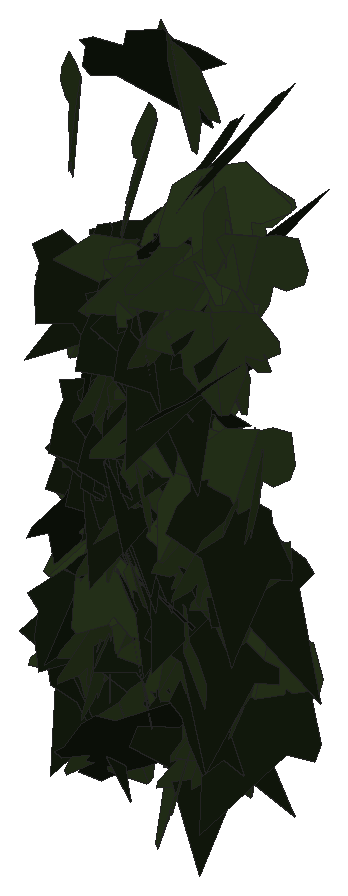
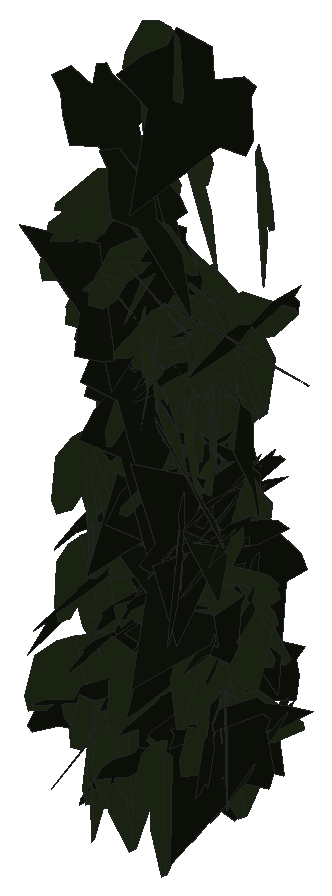
# SketchUp Ruby script. Lengths in inches.
U = 1.inch
M = Sketchup.active_model
def pt(a) = Geom::Point3d.new(a.map { |v| v * U })
def face(e, loops, mat)
  f = e.add_face(loops[0].map { |a| pt(a) })
  loops[1..].each { |l| e.add_face(l.map { |a| pt(a) }).erase! }
  f.material = f.back_material = mat if mat
  f
end
# faces: each face lists its corners as indices into pts; further lists are holes
def faces(e, pts, list, mat = nil) = list.each { |f| face(e, (f[0].is_a?(Array) ? f : [f]).map { |l| l.map { |i| pts[i] } }, mat) }
# xy, xz, yz: faces in a plane at the given z, y or x. An outline is a flat list of corners, or four numbers for a rectangle; further outlines are holes
def ring(l) = l.size == 4 ? [[l[0], l[1]], [l[2], l[1]], [l[2], l[3]], [l[0], l[3]]] : l.each_slice(2).to_a
def flat(e, list, mat, &to3) = list.each { |f| face(e, (f[0].is_a?(Array) ? f : [f]).map { |l| ring(l).map { |u, v| to3.(u, v) } }, mat) }
def xy(e, z, list, mat = nil) = flat(e, list, mat) { |x, y| [x, y, z] }
def xz(e, y, list, mat = nil) = flat(e, list, mat) { |x, z| [x, y, z] }
def yz(e, x, list, mat = nil) = flat(e, list, mat) { |y, z| [x, y, z] }
def lines(e, pts, list) = list.each { |a, b| e.add_line(pt(pts[a]), pt(pts[b])) }
# prism: a flat outline (further loops are holes) pulled along v
def prism(e, loops, v, mat = nil)
  f = face(e, loops, mat); d = Geom::Vector3d.new(v.map { |x| x * U })
  f.pushpull(f.normal.samedirection?(d) ? d.length : -d.length)
end
def box(e, o, s, mat = nil) = prism(e, [[o, [o[0] + s[0], o[1], o[2]], [o[0] + s[0], o[1] + s[1], o[2]], [o[0], o[1] + s[1], o[2]]]], [0, 0, s[2]], mat)
def at(x, y, z, deg = 0) = Geom::Transformation.translation(pt([x, y, z])) * Geom::Transformation.rotation(ORIGIN, Z_AXIS, deg.degrees)
def axes(o, x, y, z) = Geom::Transformation.new([*x, 0, *y, 0, *z, 0, *pt(o).to_a, 1])
def part(name) = M.definitions.add(name)
# library, detail: a bought-in or finely detailed component or shape, given as its bounding box
def library(name, o, s) = part(name).tap { |d| box(d.entities, o, s) }
def detail(e, o, s) = box(e.add_group.entities, o, s)
def put(e, d, t, mat = nil) = e.add_instance(d, t).tap { |i| i.material = mat if mat }
def group(e, t, mat = nil) = e.add_group.tap { |g| g.transformation = t; g.material = mat if mat }.entities
root = M.entities
M.materials.add("efeu1").color = [18, 25, 13]
M.materials.add("efeu2").color = [43, 57, 29]
c1 = part("ivyleaf_10")
p = [[0,0.5,-0.03],[-0.0625,2.02,-0.43],[-0.19,2.01,-0.46],[-0.54,1.05,-0.29],[-0.52,0.625,-0.18],[-0.83,0.76,-0.28],
  [-1.16,0.64,-0.33],[-1.15,0.33,-0.24],[-0.77,-0.39,0.02],[-0.3,-0.51,0.16],[0.04,-0.48,0.23],[-0.02,2.01,-0.4375],
  [-0.06,2.01,-0.43],[0.04,-0.49,0.23],[0.67,-0.49,0.14],[1.38,0.36,-0.2],[1.375,0.51,-0.24],[0.81,0.65,-0.19],
  [0.62,0.59,-0.15],[0.6,1.09,-0.28],[0.5,1.23,-0.31]]
faces(c1.entities,p,[[0,1,2,3,4,5,6,7,8,9,10],[11,12,0,13,14,15,16,17,18,19,20]],"efeu2")
c2 = part("ivyleaf_9")
p = [[1.54,2.16,1.25],[1.36,2.04,1.19],[-0.21,0.99,0.68],[-0.71,1.11,0.82],[-0.85,0.86,0.67],[-0.8,0.17,0.21],
  [-0.9,-0.01,0.1],[-0.67,-0.16,-0.02],[-0.08,-0.08,-0.05],[-0.03,-0.6,-0.4],[0.65,-0.88,-0.66],[0.83,-0.6,-0.49],
  [1.29,-0.42,-0.43],[1.8125,-0.07,-0.26],[1.21,0.44,0.15]]
faces(c2.entities,p,[[0,1,2,3,4,5,6,7,8,9,10,11,12,13,14]],"efeu1")
put(root,c1,axes([13.96,224.02,226.48],[-0.12869,-0.48261,0.02288],[-0.00453,-0.02247,-0.49947],[0.48313,-0.12876,0.00141]))
put(root,c2,axes([14.07,224.29,227.32],[-0.23689,-0.43392,0.07482],[0.01205,-0.09132,-0.49144],[0.44016,-0.23103,0.05372]))
put(root,c1,axes([14.31,223.89,230.38],[-0.44358,0.22112,0.06589],[-0.06998,0.00713,-0.49503],[-0.21986,-0.44839,0.02463]))
put(root,c1,axes([13.77,224.05,229.28],[0.28039,-0.4139,0.00816],[0.00734,-0.00488,-0.49992],[0.41392,0.28046,0.00334]))
put(root,c2,axes([13.1,224.04,227.85],[0.12777,-0.4541,-0.16573],[-0.03569,0.16209,-0.47165],[0.48208,0.13235,0.00901]))
put(root,c2,axes([13.4375,223.77,222.93],[0.23047,0.42069,-0.14108],[0.06968,0.12269,0.47968],[0.43821,-0.24077,-0.00207]))
put(root,c1,axes([14.66,223.95,227.68],[-0.41709,-0.27569,-0.00562],[0.0048,0.00294,-0.49997],[0.2757,-0.41712,0.00019]))
put(root,c1,axes([14.52,224.01,228.11],[-0.28727,-0.40846,0.02511],[-0.0115,-0.02262,-0.49936],[0.40907,-0.28748,0.0036]))
put(root,c1,axes([13.68,223.97,225.35],[-0.02424,-0.49206,-0.08536],[0.02223,0.08431,-0.49234],[0.49892,-0.02767,0.01779]))
put(root,c1,axes([13.62,223.91,224.78],[-0.2972,-0.28507,-0.28356],[0.29254,0.0886,-0.39569],[0.27584,-0.40111,0.11413]))
put(root,c2,axes([13.67,224.16,224.9],[-0.0708,0.26948,-0.41517],[0.0066,-0.41885,-0.27299],[-0.49492,-0.04413,0.05575]))
put(root,c1,axes([13.27,224.19,227.8125],[-0.16473,-0.43142,0.19169],[-0.02068,-0.19623,-0.45942],[0.47163,-0.15929,0.04681]))
put(root,c2,axes([13.44,224.35,225.83],[-0.17086,-0.45753,0.1071],[0.02661,-0.1232,-0.48385],[0.46915,-0.15964,0.06645]))
put(root,c2,axes([14.64,224.3,225.54],[0.00782,-0.49015,0.09847],[0.02788,-0.0979,-0.48953],[0.49916,0.01314,0.0258]))
put(root,c2,axes([13.74,224.24,227.85],[-0.49927,0.01901,0.01929],[-0.02354,-0.12868,-0.48258],[-0.01338,-0.48278,0.12939]))
put(root,c1,axes([13.96,224.04,227.91],[-0.27643,-0.41617,-0.01983],[0.02125,0.00968,-0.49945],[0.4161,-0.27697,0.01233]))
put(root,c1,axes([14.35,224.1,228.51],[0.49303,-0.08212,-0.01343],[-0.01371,-0.00055,-0.49981],[0.08207,0.49321,-0.00279]))
put(root,c1,axes([12.98,224,229.5],[0.31421,-0.36758,-0.12712],[0.00084,0.16406,-0.47232],[0.38894,0.2966,0.10371]))
put(root,c1,axes([14.14,224.12,223.02],[0.33025,-0.37539,-0.00491],[-0.00238,0.00444,-0.49997],[0.37541,0.33025,0.00114]))
put(root,c1,axes([14,224.16,227.47],[0.11055,-0.48429,0.05695],[0.04014,-0.04916,-0.49596],[0.48597,0.11423,0.02801]))
put(root,c2,axes([13.96,224.24,227.22],[0.08736,-0.49112,-0.03423],[-0.00568,0.03376,-0.49883],[0.49228,0.08754,0.00032]))
put(root,c1,axes([14.61,224.0625,225.43],[0.06692,-0.4886,-0.0824],[0.01008,0.08448,-0.49271],[0.4954,0.06428,0.02116]))
put(root,c1,axes([14.3,224.34,226.03],[-0.13339,-0.37092,0.30761],[0.04431,-0.32727,-0.37541],[0.47984,-0.07289,0.12018]))
put(root,c2,axes([13.64,224.2,227.34],[0.0323,-0.48434,-0.11988],[0.01505,0.12103,-0.4849],[0.49873,0.02771,0.0224]))
put(root,c1,axes([14.35,223.95,224.21],[-0.30761,0.21132,0.33275],[-0.34447,0.06107,-0.35722],[-0.19161,-0.44902,0.10802]))
put(root,c1,axes([13.47,224.09,226.86],[0.05529,-0.49298,-0.06252],[-0.00256,0.06262,-0.49606],[0.49693,0.05518,0.00441]))
put(root,c2,axes([13.34,224.44,225.72],[-0.00155,-0.38902,0.3141],[0.0974,-0.30832,-0.38138],[0.49042,0.06001,0.07674]))
put(root,c2,axes([14.4,223.86,226.89],[0.00022,0.49983,0.01293],[-0.08835,0.01277,-0.49197],[-0.49213,-0.00207,0.08833]))
put(root,c1,axes([13.45,224.08,226.93],[0.20109,-0.44801,-0.09407],[0.02716,0.11424,-0.48602],[0.45697,0.19036,0.07028]))
put(root,c1,axes([13.53,224.03,224.98],[-0.34659,0.36024,-0.01003],[0.00737,-0.00683,-0.4999],[-0.3603,-0.34667,-0.00058]))
put(root,c2,axes([14.99,224.04,229.78],[-0.26177,0.42181,-0.0596],[-0.0172,-0.08036,-0.4932],[-0.42565,-0.25616,0.05659]))
put(root,c2,axes([13.82,224.36,226.4],[-0.43863,-0.23831,-0.02843],[0.02647,0.01082,-0.49918],[0.23854,-0.43942,0.00313]))
put(root,c1,axes([14.53,224.11,228.96],[0.27141,0.41962,0.01595],[0.01343,0.01031,-0.49971],[-0.41971,0.27168,-0.00567]))
put(root,c2,axes([14.23,224.21,227.98],[-0.46638,0.17963,-0.0148],[0.00722,-0.02238,-0.49945],[-0.18009,-0.46608,0.01828]))
put(root,c1,axes([13.67,224.2,227.68],[0.38855,0.02237,-0.3139],[-0.31391,-0.00755,-0.3891],[-0.02215,0.49944,0.00818]))
put(root,c1,axes([14.89,224.23,228.4],[-0.29515,-0.39289,0.09233],[-0.01799,-0.10146,-0.48927],[0.40319,-0.29214,0.04575]))
put(root,c2,axes([13.15,224.33,226.13],[0.07998,-0.49265,-0.02999],[0.00117,0.03057,-0.49906],[0.49356,0.07976,0.00604]))
put(root,c2,axes([13.4375,224.38,225.875],[0.08016,-0.49036,0.05587],[0.00718,-0.05544,-0.49687],[0.49348,0.08046,-0.00185]))
put(root,c1,axes([13.51,224.05,223.22],[-0.13854,-0.44051,-0.19173],[0.06607,0.18017,-0.46171],[0.47586,-0.15327,0.00829]))
put(root,c1,axes([13.47,224.3125,226.73],[0.14858,-0.46548,0.10607],[0.01529,-0.10639,-0.48831],[0.47717,0.14835,-0.01738]))
put(root,c2,axes([13.1875,224.09,225.4375],[-0.04274,0.45849,-0.19484],[0.01645,-0.19416,-0.46047],[-0.4979,-0.04577,0.00151]))
put(root,c1,axes([13.26,224.27,224.07],[0.01556,-0.49491,0.06943],[0.00361,-0.06935,-0.49515],[0.49974,0.01591,0.00142]))
put(root,c1,axes([13.74,224.15,227.68],[-0.30903,-0.39139,-0.03631],[0.02036,0.03019,-0.49867],[0.39254,-0.30969,-0.00273]))
put(root,c2,axes([13.67,223.9375,230.27],[0.42312,0.26428,-0.0336],[-0.02926,-0.01658,-0.49887],[-0.26479,0.42413,0.00143]))
put(root,c2,axes([13.35,224.39,225.66],[0.13436,-0.47691,0.06715],[0.01556,-0.06538,-0.49546],[0.48136,0.13523,-0.00273]))
put(root,c1,axes([13.97,224.21,227.75],[-0.42998,-0.14567,0.20951],[-0.19301,-0.08288,-0.45374],[0.16692,-0.47108,0.01505]))
put(root,c2,axes([14.35,224.47,224.29],[-0.04656,-0.49265,0.07158],[0.00818,-0.07264,-0.49463],[0.49776,-0.04489,0.01482]))
put(root,c1,axes([14.03,224.27,227.64],[0.10979,-0.48765,0.01218],[0.00437,-0.0115,-0.49985],[0.48778,0.10986,0.00174]))
put(root,c1,axes([13.3,224.17,224.02],[-0.01667,-0.48998,-0.09817],[-0.0088,0.0985,-0.49012],[0.49964,-0.01461,-0.0119]))
put(root,c2,axes([12.74,224.39,223.43],[0.24666,-0.42847,0.07463],[0.03064,-0.06846,-0.49434],[0.43384,0.24844,-0.00752]))
put(root,c2,axes([13.36,224.41,225.64],[0.03521,-0.49562,-0.05584],[0.00876,0.05658,-0.49671],[0.49868,0.034,0.01267]))
put(root,c2,axes([13.75,224.54,225.02],[-0.07811,-0.48413,0.09755],[-0.02047,-0.0955,-0.49037],[0.49344,-0.0806,-0.0049]))
put(root,c2,axes([14.47,224.28,227.75],[-0.45913,0.19783,0.00784],[-0.00761,0.00217,-0.49994],[-0.19784,-0.45919,0.00102]))
put(root,c1,axes([14.24,224.21,228.2],[-0.26793,-0.41499,-0.07741],[0.05714,0.05519,-0.49365],[0.41826,-0.27338,0.01786]))
put(root,c1,axes([13.6,224.44,224.76],[-0.11463,-0.44488,0.19733],[0.01179,-0.20521,-0.4558],[0.48654,-0.09984,0.05754]))
put(root,c1,axes([13.55,224.24,227.59],[-0.23492,0.43239,-0.0886],[0.02906,-0.085,-0.49186],[-0.44042,-0.23625,0.0148]))
put(root,c2,axes([13,224.57,224.68],[0.07903,-0.29497,0.39591],[0.16466,-0.36225,-0.30276],[0.46545,0.17823,0.03989]))
put(root,c2,axes([13.09,224.54,223.72],[-0.29512,-0.40268,0.02751],[-0.00913,-0.02741,-0.49916],[0.40351,-0.29513,0.00883]))
put(root,c2,axes([13.6,224.15,224.5],[0.49507,-0.06981,0.00522],[0.00542,0.00104,-0.49997],[0.0698,0.4951,0.00179]))
put(root,c2,axes([13.08,224.21,224.3125],[-0.02934,-0.33205,-0.37267],[0.05611,0.36875,-0.33298],[0.49597,-0.06136,0.01562]))
put(root,c2,axes([13.97,224.63,224.93],[-0.12386,-0.4512,0.1763],[-0.00378,-0.18106,-0.46605],[0.4844,-0.11679,0.04144]))
put(root,c1,axes([14.18,224.45,225.11],[0.03891,-0.47503,0.1511],[0.02288,-0.1497,-0.47651],[0.49796,0.04399,0.01009]))
put(root,c1,axes([13.35,224.23,226.15],[-0.48673,-0.01853,0.11294],[-0.11284,-0.00464,-0.48708],[0.0191,-0.49964,0.00034]))
put(root,c1,axes([13.97,224.08,225.08],[-0.11981,-0.26569,-0.40627],[0.32562,0.26636,-0.27022],[0.36002,-0.32933,0.10921]))
put(root,c1,axes([13.0625,224.39,223.68],[-0.26797,-0.41416,0.08164],[0.02896,-0.11451,-0.48585],[0.42113,-0.25566,0.08536]))
put(root,c1,axes([13.46,224.32,226.04],[-0.24903,-0.43341,-0.01185],[0.04199,-0.01051,-0.49812],[0.43153,-0.24909,0.04163]))
put(root,c2,axes([14.35,224.17,229.12],[-0.25447,0.4304,-0.00083],[0.00178,0.00009,-0.5],[-0.4304,-0.25447,-0.00158]))
put(root,c2,axes([13.13,223.97,226.52],[0.01077,0.06206,0.49602],[-0.03511,0.495,-0.06117],[-0.49865,-0.03352,0.01502]))
put(root,c1,axes([13.95,224.37,225.54],[-0.22451,-0.4452,0.03732],[0.00849,-0.04601,-0.49781],[0.44668,-0.22289,0.02822]))
put(root,c1,axes([14.66,224.23,228.78],[0.027,0.49764,0.04037],[0.00399,0.04022,-0.49836],[-0.49925,0.02723,-0.0018]))
put(root,c1,axes([13.77,224.28,227.82],[0.14498,0.47834,-0.01314],[-0.00369,-0.01261,-0.49983],[-0.47851,0.14503,-0.00013]))
put(root,c1,axes([13.1875,224.21,223.79],[0.17709,-0.41075,-0.22343],[-0.03268,0.22746,-0.44407],[0.46644,0.17188,0.05372]))
put(root,c2,axes([13.19,224.53,225.67],[-0.07213,-0.48739,-0.08512],[0.04377,0.0794,-0.49171],[0.49283,-0.07839,0.03121]))
put(root,c2,axes([13.44,224.54,225.66],[0.11,-0.48696,0.02777],[0.00336,-0.02771,-0.49922],[0.48774,0.11001,-0.00283]))
put(root,c1,axes([13.69,224.18,225.91],[-0.19742,0.42277,0.17969],[-0.12327,0.13965,-0.464],[-0.44252,-0.22751,0.04909]))
put(root,c2,axes([14.36,224.13,228.38],[0.30227,0.37096,-0.14499],[-0.15566,-0.05751,-0.47166],[-0.36661,0.33028,0.08072]))
put(root,c2,axes([13.4375,224.53,225.64],[0.25236,-0.42752,0.05948],[0.02233,-0.05587,-0.49637],[0.43106,0.25318,-0.0091]))
put(root,c1,axes([14.32,224.25,228.01],[0.15494,0.461,0.11606],[0.00443,0.12066,-0.4852],[-0.47537,0.15138,0.03331]))
put(root,c1,axes([13.97,224.4,226.9375],[-0.20795,-0.45429,-0.01944],[0.03934,0.00332,-0.49844],[0.453,-0.20883,0.03436]))
put(root,c1,axes([14.61,224.52,226.15],[-0.20348,-0.43641,0.13468],[-0.00086,-0.14708,-0.47788],[0.45672,-0.19471,0.05911]))
put(root,c2,axes([13.58,224.49,226.33],[0.10613,-0.4756,-0.11197],[0.02439,0.11959,-0.48487],[0.488,0.09746,0.04859]))
put(root,c2,axes([13.07,224.42,225.74],[0.31353,-0.38518,-0.05775],[0.00548,0.0785,-0.49377],[0.38945,0.30899,0.05345]))
put(root,c2,axes([14.03,224.62,223.11],[-0.02252,-0.49942,0.00823],[-0.00634,-0.00796,-0.4999],[0.49945,-0.02262,-0.00597]))
put(root,c2,axes([14.3,224.29,223.63],[0.31332,-0.31073,-0.23512],[-0.11189,0.21725,-0.43621],[0.37325,0.32596,0.0666]))
put(root,c1,axes([13.8125,224.5,226.86],[0.38668,-0.2523,0.19188],[0.19982,-0.04093,-0.4565],[0.24606,0.42973,0.06918]))
put(root,c1,axes([14.36,224.55,223.24],[0.05365,-0.48151,0.12356],[0.01205,-0.12298,-0.48449],[0.49697,0.05496,-0.00159]))
put(root,c1,axes([14.39,224.34,227.5],[-0.48062,0.13761,-0.0084],[0.00948,0.00259,-0.4999],[-0.13754,-0.48069,-0.0051]))
put(root,c1,axes([13.94,224.55,223.96],[-0.178,-0.44183,0.15201],[-0.02433,-0.15368,-0.47517],[0.46661,-0.17655,0.03321]))
put(root,c1,axes([13.85,224.34,226.42],[-0.34659,-0.16163,-0.3221],[0.32411,0.05559,-0.37665],[0.15757,-0.46988,0.06623]))
put(root,c2,axes([13.58,224.37,226.61],[0.47391,-0.15922,-0.00772],[-0.01126,-0.00931,-0.49979],[0.15901,0.47388,-0.01241]))
put(root,c1,axes([13.18,224.56,225.08],[0.32912,0.16711,-0.33728],[-0.31081,-0.13206,-0.36872],[-0.21232,0.45236,0.01695]))
put(root,c1,axes([14.69,224.52,224.93],[-0.073,-0.49185,0.05244],[-0.01045,-0.05146,-0.49724],[0.49453,-0.07369,-0.00277]))
put(root,c1,axes([13.11,224.41,224],[0.21987,-0.43876,-0.09561],[0.03832,0.1244,-0.48276],[0.44742,0.20496,0.08833]))
put(root,c1,axes([14.33,224.49,223],[-0.09408,-0.49096,0.01044],[-0.00352,-0.00996,-0.49989],[0.49106,-0.09413,-0.00158]))
put(root,c1,axes([14.11,224.29,227.37],[-0.32638,0.3388,0.16938],[-0.13635,0.10351,-0.46978],[-0.35339,-0.35285,0.02482]))
put(root,c1,axes([13.2,224.6,225.03],[-0.24237,-0.40933,0.15396],[-0.01534,-0.16796,-0.4707],[0.43706,-0.23289,0.06885]))
put(root,c2,axes([13.69,224.18,225.92],[-0.0847,0.44084,0.2202],[-0.15345,0.18873,-0.43685],[-0.46827,-0.14158,0.10332]))
put(root,c1,axes([13.5,224.3,224.75],[0.15869,0.42807,0.20389],[0.08673,0.18517,-0.45628],[-0.46615,0.18018,-0.01549]))
put(root,c2,axes([14.62,224.76,223.55],[-0.296,-0.4023,0.0232],[0.01687,-0.04114,-0.49802],[0.40262,-0.29404,0.03793]))
put(root,c2,axes([13.16,224.58,224.87],[0.33403,-0.33013,0.17158],[0.14177,-0.10025,-0.46888],[0.34398,0.36189,0.02664]))
put(root,c1,axes([14.48,224.45,223.45],[-0.10357,-0.48033,-0.09247],[0.01031,0.09236,-0.49129],[0.48905,-0.10367,-0.00922]))
put(root,c1,axes([13.42,224.38,226.6],[-0.40497,0.28383,0.07374],[-0.06234,0.03952,-0.49452],[-0.28655,-0.40973,0.00338]))
put(root,c2,axes([13.01,224.74,223.85],[0.10465,-0.04755,-0.48661],[0.47324,-0.11517,0.11303],[-0.12284,-0.48422,0.0209]))
put(root,c1,axes([13.59,224.45,226.39],[0.37143,0.32095,0.09505],[0.05742,0.07879,-0.4904],[-0.32977,0.37521,0.02167]))
put(root,c2,axes([14.05,224.3,227.32],[0.03493,0.49876,0.00428],[0.00872,0.00368,-0.49991],[-0.4987,0.035,-0.00844]))
put(root,c1,axes([13.16,224.57,224.98],[0.40804,0.2683,-0.1073],[-0.12931,0.00351,-0.48298],[-0.25842,0.4219,0.07225]))
put(root,c2,axes([14.3,224.33,227.78],[0.06355,0.49344,-0.04981],[0.01644,0.0481,0.49741],[0.49567,-0.06486,-0.01011]))
put(root,c2,axes([13.375,224.65,224.03],[0.08648,-0.4656,-0.16042],[0.03012,0.16757,-0.47012],[0.49154,0.07164,0.05703]))
put(root,c2,axes([13.87,224.36,226.82],[0.16098,0.46614,-0.08248],[-0.02537,-0.0785,-0.49315],[-0.4727,0.16295,-0.00162]))
put(root,c1,axes([13.45,224.49,225.75],[0.12577,-0.4386,-0.20449],[0.00166,0.21167,-0.45298],[0.48392,0.11326,0.0547]))
put(root,c1,axes([14.65,224.5625,225.93],[0.28926,-0.39513,-0.10098],[0.0145,0.13369,-0.48158],[0.40758,0.27567,0.0888]))
put(root,c2,axes([13.06,224.4375,223.7],[0.42862,0.21067,-0.14801],[-0.13141,-0.06819,-0.47758],[-0.22141,0.4483,-0.00309]))
put(root,c2,axes([13.68,224.4,226.41],[0.46822,0.17216,-0.03365],[-0.04127,0.01487,-0.49807],[-0.1705,0.46919,0.02813]))
put(root,c1,axes([14.63,224.74,223.95],[-0.37588,-0.30817,0.11725],[-0.01975,-0.15644,-0.47448],[0.32913,-0.36133,0.10543]))
put(root,c1,axes([13.65,224.45,226.09],[0.0304,0.46847,0.17208],[-0.06741,0.17468,-0.46362],[-0.4945,0.00499,0.07378]))
put(root,c2,axes([14.46,224.7,224.9],[0.20056,-0.43201,-0.15212],[0.00299,0.1673,-0.47117],[0.458,0.18808,0.06969]))
put(root,c1,axes([12.92,224.57,224.93],[-0.32185,-0.09853,-0.36973],[0.36362,0.07164,-0.33563],[0.11911,-0.48493,0.02555]))
put(root,c2,axes([13.52,224.46,226.06],[0.10226,0.48667,-0.05193],[-0.01102,-0.05074,-0.4973],[-0.48931,0.10286,0.00035]))
put(root,c2,axes([13.6,224.41,226.31],[-0.14015,0.28993,0.38249],[-0.19015,0.33232,-0.32157],[-0.44068,-0.2356,0.01711]))
put(root,c2,axes([13.24,224.51,225.11],[0.4791,0.09595,-0.10607],[-0.10662,-0.00757,-0.48844],[-0.09534,0.49065,0.01321]))
put(root,c1,axes([14.41,224.69,223.21],[0.15959,-0.45164,-0.14335],[0.03606,0.1624,-0.47151],[0.47247,0.14016,0.0844]))
put(root,c2,axes([13.22,224.51,225.75],[-0.14508,-0.10801,0.46614],[0.37573,0.27588,0.18087],[-0.29627,0.40277,0.00112]))
put(root,c1,axes([13.07,224.7,224.85],[-0.31602,-0.36725,-0.12351],[0.10458,0.07262,-0.48352],[0.37308,-0.33144,0.03092]))
put(root,c2,axes([13.49,224.48,225.92],[0.06704,0.01339,-0.4953],[-0.445,0.22143,-0.05424],[0.2179,0.44809,0.04161]))
put(root,c1,axes([13.5,224.82,223.22],[-0.03465,-0.48548,-0.11451],[-0.00109,0.11486,-0.48663],[0.4988,-0.03347,-0.00902]))
put(root,c2,axes([13.29,224.53,225.2],[0.20285,0.39667,0.22694],[0.01351,0.24299,-0.43678],[-0.4568,0.18333,0.08786]))
